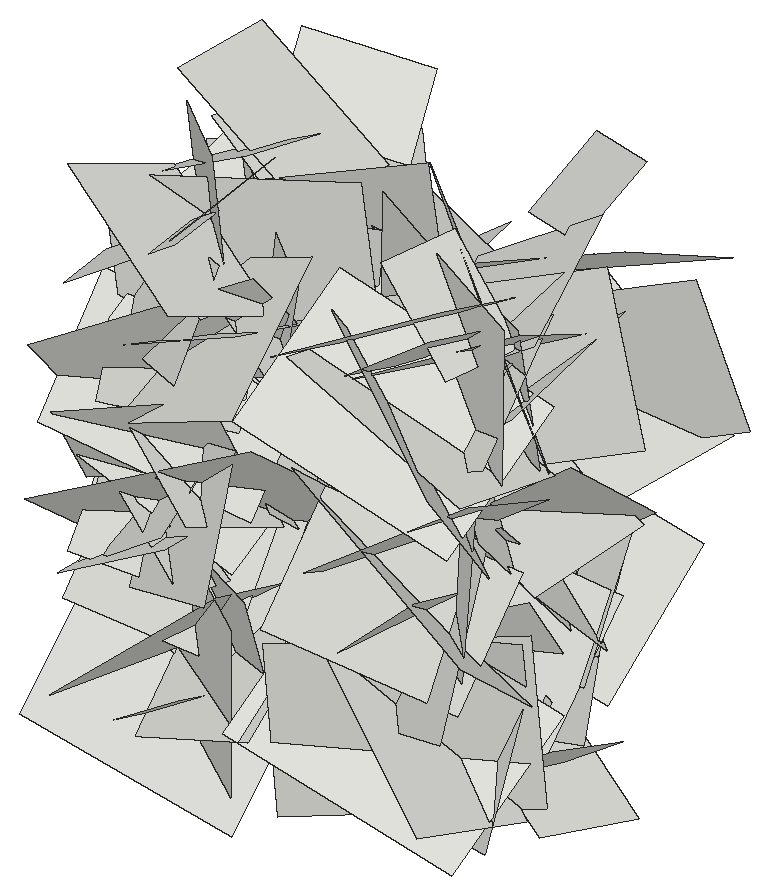
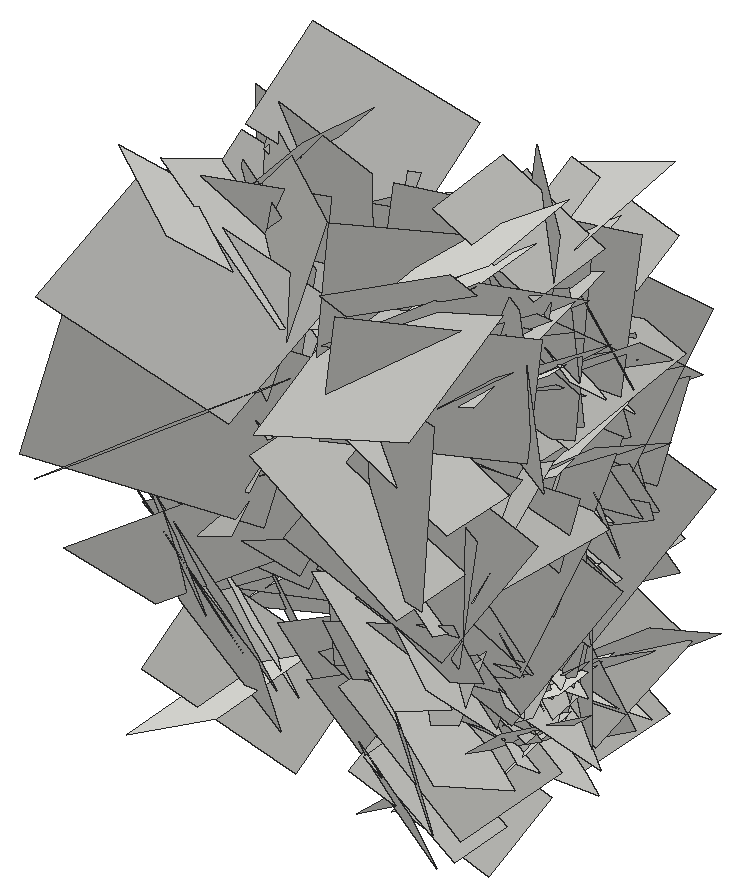
# SketchUp Ruby script. Lengths in inches.
U = 1.inch
M = Sketchup.active_model
def pt(a) = Geom::Point3d.new(a.map { |v| v * U })
def face(e, loops, mat)
  f = e.add_face(loops[0].map { |a| pt(a) })
  loops[1..].each { |l| e.add_face(l.map { |a| pt(a) }).erase! }
  f.material = f.back_material = mat if mat
  f
end
# faces: each face lists its corners as indices into pts; further lists are holes
def faces(e, pts, list, mat = nil) = list.each { |f| face(e, (f[0].is_a?(Array) ? f : [f]).map { |l| l.map { |i| pts[i] } }, mat) }
# xy, xz, yz: faces in a plane at the given z, y or x. An outline is a flat list of corners, or four numbers for a rectangle; further outlines are holes
def ring(l) = l.size == 4 ? [[l[0], l[1]], [l[2], l[1]], [l[2], l[3]], [l[0], l[3]]] : l.each_slice(2).to_a
def flat(e, list, mat, &to3) = list.each { |f| face(e, (f[0].is_a?(Array) ? f : [f]).map { |l| ring(l).map { |u, v| to3.(u, v) } }, mat) }
def xy(e, z, list, mat = nil) = flat(e, list, mat) { |x, y| [x, y, z] }
def xz(e, y, list, mat = nil) = flat(e, list, mat) { |x, z| [x, y, z] }
def yz(e, x, list, mat = nil) = flat(e, list, mat) { |y, z| [x, y, z] }
def lines(e, pts, list) = list.each { |a, b| e.add_line(pt(pts[a]), pt(pts[b])) }
# prism: a flat outline (further loops are holes) pulled along v
def prism(e, loops, v, mat = nil)
  f = face(e, loops, mat); d = Geom::Vector3d.new(v.map { |x| x * U })
  f.pushpull(f.normal.samedirection?(d) ? d.length : -d.length)
end
def box(e, o, s, mat = nil) = prism(e, [[o, [o[0] + s[0], o[1], o[2]], [o[0] + s[0], o[1] + s[1], o[2]], [o[0], o[1] + s[1], o[2]]]], [0, 0, s[2]], mat)
def at(x, y, z, deg = 0) = Geom::Transformation.translation(pt([x, y, z])) * Geom::Transformation.rotation(ORIGIN, Z_AXIS, deg.degrees)
def axes(o, x, y, z) = Geom::Transformation.new([*x, 0, *y, 0, *z, 0, *pt(o).to_a, 1])
def part(name) = M.definitions.add(name)
# library, detail: a bought-in or finely detailed component or shape, given as its bounding box
def library(name, o, s) = part(name).tap { |d| box(d.entities, o, s) }
def detail(e, o, s) = box(e.add_group.entities, o, s)
def put(e, d, t, mat = nil) = e.add_instance(d, t).tap { |i| i.material = mat if mat }
def group(e, t, mat = nil) = e.add_group.tap { |g| g.transformation = t; g.material = mat if mat }.entities
root = M.entities
c1 = part("Component\#6")
p = [[0.01,0,0],[0,3.24,4.54],[4.32,3.24,4.54],[4.33,0,0]]
faces(c1.entities,p,[[0,1,2,3]])
put(root,c1,axes([24.34,139.47,36.72],[0.15825,-0.66033,0.08813],[0.02764,0.09604,0.67542],[0.70562,0.14433,-0.04622]))
put(root,c1,axes([28.31,137.53,34.5],[0.08019,0.3809,0.76753],[-0.04804,0.77121,-0.37826],[-0.90698,-0.00717,0.08789]))
put(root,c1,axes([28.31,137.14,29.31],[-0.00249,0.75761,-0.01469],[-0.08098,-0.01485,-0.75375],[-0.79913,-0.00085,0.07643]))
put(root,c1,axes([28.31,149.44,28.46],[0.01637,-0.35652,-0.61871],[-0.18604,-0.60176,0.34238],[-0.7337,0.14463,-0.10062]))
put(root,c1,axes([24.34,144.76,23.61],[0.10873,-0.7568,0.02149],[-0.01122,0.02025,0.76368],[0.80245,0.10283,0.00777]))
put(root,c1,axes([28.31,139.84,37.375],[-0.13047,0.02824,0.77],[0.11824,0.77221,-0.01049],[-0.80815,0.10842,-0.12584]))
put(root,c1,axes([24.34,147.86,21.63],[-0.08807,-1.00346,0.13322],[-0.11481,0.14172,0.99989],[1.06685,-0.06759,0.1186]))
put(root,c1,axes([24.34,145.6875,25.3],[-0.21495,-0.77208,-0.77151],[-0.06755,-0.77499,0.79232],[1.15499,-0.18901,-0.09724]))
put(root,c1,axes([24.34,141.61,27.46],[-0.15544,0.8369,-0.58263],[-0.03072,-0.5918,-0.84279],[1.08048,0.10358,-0.10778]))
put(root,c1,axes([28.31,146.7,34.04],[0.22474,0.77203,-0.6543],[0.03576,-0.67353,-0.78378],[-1.07212,0.13937,-0.1633]))
put(root,c1,axes([28.31,140.76,35.5625],[-0.0095,0.80566,-0.00603],[0.04784,-0.00552,-0.80445],[-0.85268,-0.00929,-0.04507]))
put(root,c1,axes([28.31,144.98,23.12],[-0.11015,0.70988,0.06167],[0.04855,0.06885,-0.71532],[-0.75374,-0.09931,-0.05509]))
put(root,c1,axes([24.34,147.08,31.53],[-0.0186,0.21399,-0.90436],[-0.04027,-0.90393,-0.21315],[0.98427,-0.03294,-0.02581]))
put(root,c1,axes([24.34,137.85,30.84],[-0.06669,0.91948,0.38333],[-0.06841,0.37952,-0.92095],[1.05374,0.08283,-0.03553]))
put(root,c1,axes([28.31,143.64,28.51],[-0.01569,-0.00258,-0.72773],[-0.02057,-0.72762,0.00297],[-0.77112,0.01947,0.01473]))
put(root,c1,axes([24.34,144.71,33.13],[-0.16995,0.04512,1.05289],[-0.00982,1.0649,-0.04705],[1.11704,0.01623,0.15977]))
put(root,c1,axes([24.34,149.13,24.11],[-0.03147,-0.85153,-0.39996],[-0.02133,-0.3995,0.85202],[0.997,-0.03542,0.00561]))
put(root,c1,axes([24.34,150.98,27.43],[0.11329,-0.77541,-0.3635],[-0.07754,-0.37325,0.77469],[0.90445,0.06513,0.11195]))
put(root,c1,axes([24.34,138.53,29.67],[0.03677,-0.4198,0.69058],[0.10131,0.68849,0.41374],[0.85065,-0.06385,-0.07912]))
put(root,c1,axes([28.31,144.05,31.85],[0.11078,0.17753,-0.74918],[-0.12323,-0.74375,-0.19246],[-0.80677,0.13798,-0.07348]))
put(root,c1,axes([28.31,143.38,25.93],[0.00088,-0.66729,0.07011],[-0.1194,0.06898,0.65784],[-0.70113,-0.01259,-0.11194]))
put(root,c1,axes([28.31,140.84,40.56],[0.05261,0.712,-0.12967],[-0.10362,-0.12219,-0.70833],[-0.7601,0.06594,0.08758]))
put(root,c1,axes([24.34,148.52,32.35],[0.08011,-0.79067,-0.06214],[0.07476,-0.05548,0.79163],[0.83736,0.0806,-0.06473]))
put(root,c1,axes([24.34,142.67,41.25],[-0.05619,0.9574,-0.08237],[0.00834,-0.08206,-0.95886],[1.01856,0.05349,0.00331]))
put(root,c1,axes([28.31,144.6,22.65],[0.17478,-0.82558,-0.09028],[-0.09417,-0.10904,0.83495],[-0.87528,-0.15312,-0.10786]))
put(root,c1,axes([24.34,145.42,24.52],[-0.2647,-0.88765,0.75819],[-0.01358,0.77738,0.90589],[1.23735,-0.18136,0.17214]))
put(root,c1,axes([24.34,141.63,23.18],[-0.01995,1.00092,0.30572],[-0.13829,0.30114,-0.99396],[1.10071,0.05598,-0.11933]))
put(root,c1,axes([28.31,145.6,27.28],[-0.00806,0.29423,-0.56577],[-0.12293,-0.55701,-0.28812],[-0.6647,0.09945,0.06014]))
put(root,c1,axes([24.34,135.48,23.28],[-0.21581,1.04519,0.5846],[-0.09636,0.57779,-1.06467],[1.26577,0.22219,0.01862]))
put(root,c1,axes([28.31,143.53,22.21],[0.15224,-0.84766,-0.36991],[0.10957,-0.35729,0.85887],[-0.97421,-0.17265,0.03879]))
put(root,c1,axes([28.31,137.77,24.11],[0.1419,0.78136,-0.16109],[-0.04598,-0.15597,-0.79258],[-0.84441,0.13979,0.01609]))
put(root,c1,axes([24.34,136.3,32.46],[-0.17238,0.91042,0.71253],[-0.07022,0.71102,-0.92361],[1.22345,0.16908,0.04738]))
put(root,c1,axes([24.34,137.68,27.62],[0.00267,0.49736,0.77514],[0.05686,0.77375,-0.49665],[0.97459,-0.04651,0.02685]))
put(root,c1,axes([24.34,145.12,23.07],[-0.0526,-0.82286,-0.58821],[0.0059,-0.58914,0.82367],[1.07215,-0.03713,-0.03339]))
put(root,c1,axes([28.31,145.7,22.51],[0.08358,0.19729,0.79599],[0.0899,0.79341,-0.20506],[-0.86462,0.10156,0.05562]))
put(root,c1,axes([28.31,146.3,23.53],[0.0913,-0.50535,0.50896],[-0.05568,0.5068,0.51209],[-0.75823,-0.09807,0.02368]))
put(root,c1,axes([28.31,145.72,37.21],[-0.0202,-0.65006,0.07365],[0.02062,0.07308,0.65011],[-0.69316,0.02112,0.01719]))
put(root,c1,axes([28.31,141.16,33.73],[-0.01034,-0.20439,-0.70125],[0.11317,-0.69418,0.20085],[-0.76594,-0.09981,0.03914]))
put(root,c1,axes([24.34,149.17,29.19],[0.22051,-0.77582,-0.34275],[-0.07369,-0.36732,0.78924],[0.89602,0.16072,0.14925]))
put(root,c1,axes([28.31,144.18,33.46],[0.08879,-0.56105,-0.39599],[-0.0694,-0.40364,0.55803],[-0.72461,-0.03009,-0.10197]))
put(root,c1,axes([28.31,136.92,29.78],[-0.03864,0.57092,0.32429],[0.05823,0.3263,-0.56829],[-0.69355,-0.00442,-0.06578]))
put(root,c1,axes([28.31,146.45,21.25],[0.00375,0.2874,0.54008],[-0.0654,0.5375,-0.28562],[-0.64519,-0.05282,0.03209]))
put(root,c1,axes([28.31,144.73,33.27],[0.16555,-0.76551,-0.15352],[-0.02389,-0.16091,0.77946],[-0.82725,-0.14855,-0.05323]))
put(root,c1,axes([24.34,144.65,25.96],[0.15377,0.53431,0.65108],[0.06081,0.65286,-0.54856],[0.89071,-0.13681,-0.07495]))
put(root,c1,axes([28.31,139.71,39.61],[-0.08624,0.67106,-0.00672],[0.16105,0.01183,-0.6586],[-0.69289,-0.08077,-0.15225]))
put(root,c1,axes([24.34,143.41,32.67],[-0.00295,0.89075,-0.72818],[-0.15415,-0.72261,-0.88339],[1.20976,-0.08991,-0.11434]))
put(root,c1,axes([24.34,146.5,19.86],[0.14062,-0.87102,0.18651],[0.03259,0.19294,0.87915],[0.94365,0.12313,-0.05815]))
put(root,c1,axes([24.34,145.05,38.54],[-0.26561,0.06521,-1.32838],[-0.06869,-1.35074,-0.05408],[1.4081,-0.05359,-0.25321]))
put(root,c1,axes([24.34,142.58,23.75],[0.11698,0.88265,-0.34817],[-0.00423,-0.35009,-0.88876],[1.00576,-0.10414,0.03675]))
put(root,c1,axes([24.34,141.41,21.99],[0.04242,-1.10503,0.33762],[-0.18816,0.32793,1.09436],[1.21025,0.08972,0.15831]))
put(root,c1,axes([28.31,145.49,24.46],[0.14807,-0.32942,-0.64401],[-0.00647,-0.65643,0.33444],[-0.76675,-0.05808,-0.12719]))
put(root,c1,axes([24.34,138.75,33.42],[0.07987,0.93748,-0.3836],[-0.04246,-0.3816,-0.94046],[1.07286,-0.0849,-0.00867]))
put(root,c1,axes([28.31,142.8,24.59],[0.06246,-0.31977,0.5346],[-0.03506,0.53462,0.32343],[-0.65938,-0.05871,0.03344]))
put(root,c1,axes([28.31,142.28,27.34],[0.09885,-0.42767,0.49172],[-0.03253,0.4933,0.43487],[-0.69002,-0.08452,0.04994]))
put(root,c1,axes([24.34,139.49,21.74],[0.04906,0.46783,0.90513],[0.0041,0.90598,-0.46846],[1.08001,-0.02469,-0.03934]))
put(root,c1,axes([28.31,149.12,29.1],[0.10824,-0.19319,-0.65872],[0.02698,-0.66445,0.19881],[-0.72715,-0.05341,-0.09068]))
put(root,c1,axes([24.34,145.04,25.97],[-0.0145,-0.85349,0.83598],[-0.13626,0.83223,0.84756],[1.25903,0.08024,0.10136]))
put(root,c1,axes([28.31,141.05,35.76],[0.06877,-0.60814,0.14272],[0.00885,0.14432,0.61116],[-0.66208,-0.06124,0.02299]))
put(root,c1,axes([28.31,149.56,39.6],[0.17317,-0.50739,-0.45031],[-0.03865,-0.46908,0.51531],[-0.71806,-0.09712,-0.13634]))
put(root,c1,axes([28.31,140.39,26.94],[0.03872,-0.62994,0.14227],[0.11345,0.14643,0.62088],[-0.67508,-0.01152,0.1125]))
put(root,c1,axes([28.31,144.97,35.07],[0.07722,-0.5315,-0.34657],[0.05738,-0.34237,0.53643],[-0.67013,-0.09056,0.006]))
put(root,c1,axes([24.34,139.67,30.68],[-0.09112,-0.77438,0.96294],[-0.03313,0.96632,0.77431],[1.3094,-0.02944,0.0866]))
put(root,c1,axes([24.34,138.43,27.8],[0.10648,0.28124,1.16655],[-0.16097,1.1642,-0.2676],[1.26174,0.12479,-0.13259]))
put(root,c1,axes([24.34,140.69,35.43],[0.02714,1.22478,0.26938],[-0.1382,0.27058,-1.21783],[1.3221,0.00314,-0.13283]))
put(root,c1,axes([24.34,137.65,40.3125],[0.15365,0.92766,-0.3555],[0.07441,-0.36793,-0.93147],[1.05042,-0.10963,0.11798]))
put(root,c1,axes([24.34,149.09,36.34],[-0.1737,0.35213,-1.24285],[0.08,-1.24806,-0.36356],[1.36694,0.11779,-0.13666]))
put(root,c1,axes([24.34,146.73,29.36],[-0.09029,-1.26195,0.03468],[0.03892,0.03227,1.26436],[1.33761,-0.08612,-0.03444]))
put(root,c1,axes([24.34,141.99,33.2],[0.15631,-0.03731,1.01998],[0.08418,1.02787,0.02612],[1.07863,-0.07482,-0.14985]))
put(root,c1,axes([24.34,141.2,30.22],[0.14348,-0.5033,-0.91823],[0.06175,-0.92081,0.51331],[1.10823,0.11647,0.09028]))
put(root,c1,axes([24.34,143.42,27.33],[0.08667,-0.86973,1.01008],[-0.23887,0.9884,0.86929],[1.39256,0.22367,0.08625]))
put(root,c1,axes([24.34,142.6875,32.73],[-0.11413,-1.14483,0.29443],[0.2702,0.26621,1.12831],[1.22353,-0.16558,-0.2217]))
put(root,c1,axes([24.34,143.97,23.32],[0.18437,0.48358,0.83906],[0.16998,0.82633,-0.50949],[1.01237,-0.22682,-0.06726]))
put(root,c1,axes([24.34,144,25.2],[0.04504,0.58566,0.95802],[0.11757,0.95183,-0.5868],[1.18441,-0.11675,0.02182]))
put(root,c1,axes([24.34,150.86,30.47],[0.14962,-1.13409,-0.09371],[-0.03493,-0.09847,1.14197],[1.20573,0.13788,0.04471]))
put(root,c1,axes([24.34,141.59,27.99],[-0.06396,0.08339,-1.32201],[-0.02487,-1.32324,-0.0824],[1.4039,-0.01964,-0.06169]))
put(root,c1,axes([24.34,145.76,27.48],[0.11303,-0.66031,-0.96553],[-0.02355,-0.9705,0.66125],[1.23968,0.04176,0.1006]))
put(root,c1,axes([24.34,149.48,27.53],[0.05839,-0.93868,-0.8352],[-0.07486,-0.83699,0.93604],[1.32974,-0.0059,0.08937]))
put(root,c1,axes([24.34,141.72,37.36],[0.19445,0.97106,0.50245],[-0.00165,0.50971,-0.98451],[1.15895,-0.1622,-0.0857]))
put(root,c1,axes([24.34,141.71,25.57],[-0.24627,-1.07768,0.84944],[0.21085,0.82598,1.10232],[1.43917,-0.30542,-0.01615]))
put(root,c1,axes([24.34,141.15,27.9],[0.10356,0.25866,-1.08582],[0.18317,-1.08033,-0.24181],[1.16891,0.14638,0.13409]))
put(root,c1,axes([24.34,145.83,38.68],[-0.04371,1.09164,-0.51046],[0.28885,-0.48908,-1.06793],[1.24431,0.15188,0.22998]))
put(root,c1,axes([24.34,140.25,33.3],[-0.10371,-0.10781,1.29757],[0.22808,1.282,0.12274],[1.36119,-0.22303,0.07829]))
put(root,c1,axes([24.34,139.39,34.34],[0.15089,0.92592,0.71699],[0.08883,0.71236,-0.93659],[1.23815,-0.16395,-0.02018]))
put(root,c1,axes([24.34,142.42,32.89],[0.18672,-0.42722,1.28431],[-0.1337,1.28432,0.44452],[1.42847,0.17605,-0.12627]))
put(root,c1,axes([24.34,142.63,35.02],[0.11092,-0.98462,-0.77371],[0.1183,-0.76598,0.98988],[1.32209,0.15114,-0.02366]))
put(root,c1,axes([24.34,137.42,26.21],[0.14568,0.69276,1.17725],[0.03045,1.18146,-0.69859],[1.44759,-0.09457,-0.10377]))
put(root,c1,axes([24.34,143.09,24.72],[0.05768,-1.1082,-0.74759],[0.23067,-0.73089,1.09928],[1.3981,0.16631,-0.15052]))
put(root,c1,axes([24.34,141,38.04],[0.14868,1.2474,-0.57055],[0.09146,-0.58042,-1.24775],[1.45112,-0.09122,0.1371]))
put(root,c1,axes([38.11,141,38.04],[-0.14868,1.2474,-0.57055],[-0.09146,-0.58042,-1.24775],[-1.45112,-0.09122,0.1371]))
put(root,c1,axes([38.11,143.09,24.72],[-0.05768,-1.1082,-0.74759],[-0.23067,-0.73089,1.09928],[-1.3981,0.16631,-0.15052]))
put(root,c1,axes([38.11,137.42,26.21],[-0.14568,0.69276,1.17725],[-0.03045,1.18146,-0.69859],[-1.44759,-0.09457,-0.10377]))
put(root,c1,axes([38.11,142.63,35.02],[-0.11092,-0.98462,-0.77371],[-0.1183,-0.76598,0.98988],[-1.32209,0.15114,-0.02366]))
put(root,c1,axes([38.11,142.42,32.89],[-0.18672,-0.42722,1.28431],[0.1337,1.28432,0.44452],[-1.42847,0.17605,-0.12627]))
put(root,c1,axes([38.11,139.39,34.34],[-0.15089,0.92592,0.71699],[-0.08883,0.71236,-0.93659],[-1.23815,-0.16395,-0.02018]))
put(root,c1,axes([38.11,140.25,33.3],[0.10371,-0.10781,1.29757],[-0.22808,1.282,0.12274],[-1.36119,-0.22303,0.07829]))
put(root,c1,axes([38.11,145.83,38.68],[0.04371,1.09164,-0.51046],[-0.28885,-0.48908,-1.06793],[-1.24431,0.15188,0.22998]))
put(root,c1,axes([38.11,141.15,27.9],[-0.10356,0.25866,-1.08582],[-0.18317,-1.08033,-0.24181],[-1.16891,0.14638,0.13409]))
put(root,c1,axes([38.11,141.71,25.57],[0.24627,-1.07768,0.84944],[-0.21085,0.82598,1.10232],[-1.43917,-0.30542,-0.01615]))
put(root,c1,axes([38.11,141.72,37.36],[-0.19445,0.97106,0.50245],[0.00165,0.50971,-0.98451],[-1.15895,-0.1622,-0.0857]))
put(root,c1,axes([38.11,149.48,27.53],[-0.05839,-0.93868,-0.8352],[0.07486,-0.83699,0.93604],[-1.32974,-0.0059,0.08937]))
put(root,c1,axes([38.11,145.76,27.48],[-0.11303,-0.66031,-0.96553],[0.02355,-0.9705,0.66125],[-1.23968,0.04176,0.1006]))
put(root,c1,axes([38.11,141.59,27.99],[0.06396,0.08339,-1.32201],[0.02487,-1.32324,-0.0824],[-1.4039,-0.01964,-0.06169]))
put(root,c1,axes([38.11,150.86,30.47],[-0.14962,-1.13409,-0.09371],[0.03493,-0.09847,1.14197],[-1.20573,0.13788,0.04471]))
put(root,c1,axes([38.11,144,25.2],[-0.04504,0.58566,0.95802],[-0.11757,0.95183,-0.5868],[-1.18441,-0.11675,0.02182]))
put(root,c1,axes([38.11,143.97,23.32],[-0.18437,0.48358,0.83906],[-0.16998,0.82633,-0.50949],[-1.01237,-0.22682,-0.06726]))
put(root,c1,axes([38.11,142.6875,32.73],[0.11413,-1.14483,0.29443],[-0.2702,0.26621,1.12831],[-1.22353,-0.16558,-0.2217]))
put(root,c1,axes([38.11,143.42,27.33],[-0.08667,-0.86973,1.01008],[0.23887,0.9884,0.86929],[-1.39256,0.22367,0.08625]))
put(root,c1,axes([38.11,141.2,30.22],[-0.14348,-0.5033,-0.91823],[-0.06175,-0.92081,0.51331],[-1.10823,0.11647,0.09028]))
put(root,c1,axes([38.11,141.99,33.2],[-0.15631,-0.03731,1.01998],[-0.08418,1.02787,0.02612],[-1.07863,-0.07482,-0.14985]))
put(root,c1,axes([38.11,146.73,29.36],[0.09029,-1.26195,0.03468],[-0.03892,0.03227,1.26436],[-1.33761,-0.08612,-0.03444]))
put(root,c1,axes([38.11,149.09,36.34],[0.1737,0.35213,-1.24285],[-0.08,-1.24806,-0.36356],[-1.36694,0.11779,-0.13666]))
put(root,c1,axes([38.11,137.65,40.3125],[-0.15365,0.92766,-0.3555],[-0.07441,-0.36793,-0.93147],[-1.05042,-0.10963,0.11798]))
put(root,c1,axes([38.11,140.69,35.43],[-0.02714,1.22478,0.26938],[0.1382,0.27058,-1.21783],[-1.3221,0.00314,-0.13283]))
put(root,c1,axes([38.11,138.43,27.8],[-0.10648,0.28124,1.16655],[0.16097,1.1642,-0.2676],[-1.26174,0.12479,-0.13259]))
put(root,c1,axes([38.11,139.67,30.68],[0.09112,-0.77438,0.96294],[0.03313,0.96632,0.77431],[-1.3094,-0.02944,0.0866]))
put(root,c1,axes([34.14,144.97,35.07],[-0.07722,-0.5315,-0.34657],[-0.05738,-0.34237,0.53643],[0.67013,-0.09056,0.006]))
put(root,c1,axes([34.14,140.39,26.94],[-0.03872,-0.62994,0.14227],[-0.11345,0.14643,0.62088],[0.67508,-0.01152,0.1125]))
put(root,c1,axes([34.14,149.56,39.6],[-0.17317,-0.50739,-0.45031],[0.03865,-0.46908,0.51531],[0.71806,-0.09712,-0.13634]))
put(root,c1,axes([34.14,141.05,35.76],[-0.06877,-0.60814,0.14272],[-0.00885,0.14432,0.61116],[0.66208,-0.06124,0.02299]))
put(root,c1,axes([38.11,145.04,25.97],[0.0145,-0.85349,0.83598],[0.13626,0.83223,0.84756],[-1.25903,0.08024,0.10136]))
put(root,c1,axes([34.14,149.12,29.1],[-0.10824,-0.19319,-0.65872],[-0.02698,-0.66445,0.19881],[0.72715,-0.05341,-0.09068]))
put(root,c1,axes([38.11,139.49,21.74],[-0.04906,0.46783,0.90513],[-0.0041,0.90598,-0.46846],[-1.08001,-0.02469,-0.03934]))
put(root,c1,axes([34.14,142.28,27.34],[-0.09885,-0.42767,0.49172],[0.03253,0.4933,0.43487],[0.69002,-0.08452,0.04994]))
put(root,c1,axes([34.14,142.8,24.59],[-0.06246,-0.31977,0.5346],[0.03506,0.53462,0.32343],[0.65938,-0.05871,0.03344]))
put(root,c1,axes([38.11,138.75,33.42],[-0.07987,0.93748,-0.3836],[0.04246,-0.3816,-0.94046],[-1.07286,-0.0849,-0.00867]))
put(root,c1,axes([34.14,145.49,24.46],[-0.14807,-0.32942,-0.64401],[0.00647,-0.65643,0.33444],[0.76675,-0.05808,-0.12719]))
put(root,c1,axes([38.11,141.41,21.99],[-0.04242,-1.10503,0.33762],[0.18816,0.32793,1.09436],[-1.21025,0.08972,0.15831]))
put(root,c1,axes([38.11,142.58,23.75],[-0.11698,0.88265,-0.34817],[0.00423,-0.35009,-0.88876],[-1.00576,-0.10414,0.03675]))
put(root,c1,axes([38.11,145.05,38.54],[0.26561,0.06521,-1.32838],[0.06869,-1.35074,-0.05408],[-1.4081,-0.05359,-0.25321]))
put(root,c1,axes([38.11,146.5,19.86],[-0.14062,-0.87102,0.18651],[-0.03259,0.19294,0.87915],[-0.94365,0.12313,-0.05815]))
put(root,c1,axes([38.11,143.41,32.67],[0.00295,0.89075,-0.72818],[0.15415,-0.72261,-0.88339],[-1.20976,-0.08991,-0.11434]))
put(root,c1,axes([34.14,139.71,39.61],[0.08624,0.67106,-0.00672],[-0.16105,0.01183,-0.6586],[0.69289,-0.08077,-0.15225]))
put(root,c1,axes([38.11,144.65,25.96],[-0.15377,0.53431,0.65108],[-0.06081,0.65286,-0.54856],[-0.89071,-0.13681,-0.07495]))
